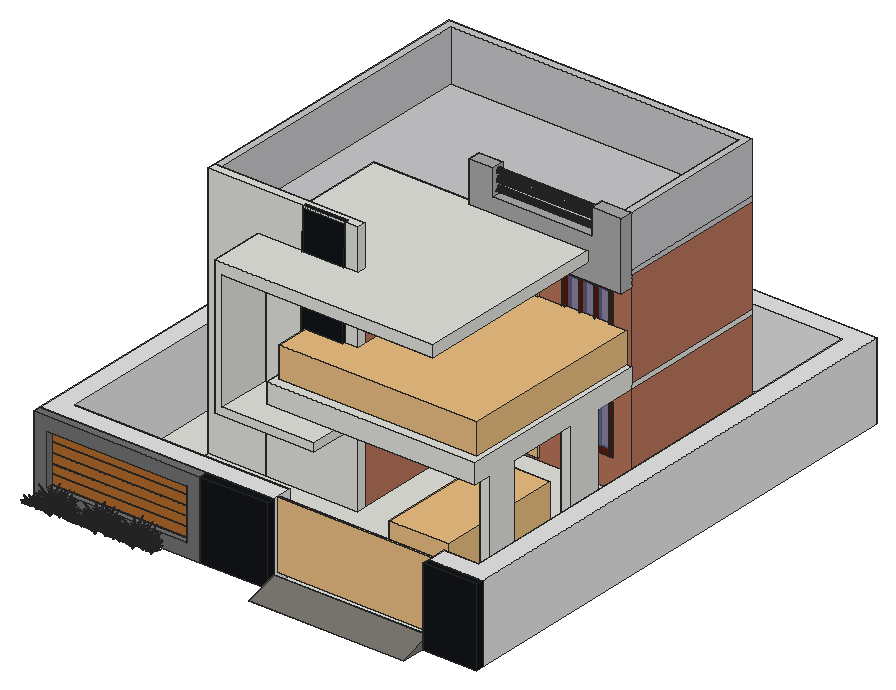
# SketchUp Ruby script. Lengths in inches.
U = 1.inch
M = Sketchup.active_model
def pt(a) = Geom::Point3d.new(a.map { |v| v * U })
def face(e, loops, mat)
  f = e.add_face(loops[0].map { |a| pt(a) })
  loops[1..].each { |l| e.add_face(l.map { |a| pt(a) }).erase! }
  f.material = f.back_material = mat if mat
  f
end
# faces: each face lists its corners as indices into pts; further lists are holes
def faces(e, pts, list, mat = nil) = list.each { |f| face(e, (f[0].is_a?(Array) ? f : [f]).map { |l| l.map { |i| pts[i] } }, mat) }
# xy, xz, yz: faces in a plane at the given z, y or x. An outline is a flat list of corners, or four numbers for a rectangle; further outlines are holes
def ring(l) = l.size == 4 ? [[l[0], l[1]], [l[2], l[1]], [l[2], l[3]], [l[0], l[3]]] : l.each_slice(2).to_a
def flat(e, list, mat, &to3) = list.each { |f| face(e, (f[0].is_a?(Array) ? f : [f]).map { |l| ring(l).map { |u, v| to3.(u, v) } }, mat) }
def xy(e, z, list, mat = nil) = flat(e, list, mat) { |x, y| [x, y, z] }
def xz(e, y, list, mat = nil) = flat(e, list, mat) { |x, z| [x, y, z] }
def yz(e, x, list, mat = nil) = flat(e, list, mat) { |y, z| [x, y, z] }
def lines(e, pts, list) = list.each { |a, b| e.add_line(pt(pts[a]), pt(pts[b])) }
# prism: a flat outline (further loops are holes) pulled along v
def prism(e, loops, v, mat = nil)
  f = face(e, loops, mat); d = Geom::Vector3d.new(v.map { |x| x * U })
  f.pushpull(f.normal.samedirection?(d) ? d.length : -d.length)
end
def box(e, o, s, mat = nil) = prism(e, [[o, [o[0] + s[0], o[1], o[2]], [o[0] + s[0], o[1] + s[1], o[2]], [o[0], o[1] + s[1], o[2]]]], [0, 0, s[2]], mat)
def at(x, y, z, deg = 0) = Geom::Transformation.translation(pt([x, y, z])) * Geom::Transformation.rotation(ORIGIN, Z_AXIS, deg.degrees)
def axes(o, x, y, z) = Geom::Transformation.new([*x, 0, *y, 0, *z, 0, *pt(o).to_a, 1])
def part(name) = M.definitions.add(name)
# library, detail: a bought-in or finely detailed component or shape, given as its bounding box
def library(name, o, s) = part(name).tap { |d| box(d.entities, o, s) }
def detail(e, o, s) = box(e.add_group.entities, o, s)
def put(e, d, t, mat = nil) = e.add_instance(d, t).tap { |i| i.material = mat if mat }
def group(e, t, mat = nil) = e.add_group.tap { |g| g.transformation = t; g.material = mat if mat }.entities
root = M.entities
M.materials.add("Teddy_HairLight").color = [51, 36, 26]
M.materials.add("[Color B08]").color = [102, 25, 0]
M.materials.add("[Color M03]").color = [170, 170, 170]
M.materials.add("[Color M05]").color = [114, 114, 114]
M.materials.add("[Color M08]").color = [30, 30, 30]
M.materials.add("[Iris]").color = [93, 63, 112]
M.materials.add("[Metal Rusted]").color = [184, 117, 91]
M.materials.add("[Polished Concrete New]").color = [200, 200, 203]
M.materials.add("[Polished Concrete Old]").color = [229, 229, 229]
M.materials.add("[Rough Square Concrete Block]").color = [123, 120, 113]
M.materials.add("[Stone Coursed Rough]").color = [19, 22, 25]
M.materials.add("[Translucent Glass Blue]").color = [100, 149, 237]
M.materials["[Translucent Glass Blue]"].alpha = 0.5
M.materials.add("[Wood Bamboo]").color = [177, 105, 43]
M.materials.add("[Wood Veneer 01]").color = [120, 70, 37]
c1 = library("Passenger sedan",[0.01,0.03,0.02],[16.17,34.46,10.62])
c2 = library("Untitled",[332.1875,126.3,0],[192,3,60])
c3 = part("Group\#23")
p = [[2.875,6.8,1.42],[2.44,3.34,0.98],[2.875,0,0],[3.31,3.34,0.98],[2.875,82.68,0],[2.44,79.33,0.98],
  [2.875,75.875,1.42],[3.31,79.33,0.98],[2,6.6875,1.96],[3.74,6.6875,1.96],[2,75.99,1.96],[3.74,75.99,1.96],
  [1.64,10.09,2.76],[4.09,10.09,2.76],[2.875,13.65,2.58],[1.64,72.59,2.76],[2.875,69.03,2.58],[4.09,72.59,2.76],
  [1.29,13.48,3.57],[4.44,13.49,3.57],[1,16.93,4.2],[4.72,16.93,4.2],[2.875,20.54,3.48],[1,65.75,4.2],
  [2.875,62.14,3.48],[4.72,65.75,4.2],[4.44,69.19,3.57],[1.29,69.19,3.57],[0.72,20.37,4.82],[5,20.37,4.82],
  [0.52,23.85,5.28],[5.19,23.85,5.28],[2.875,27.46,4.13],[0.52,58.83,5.28],[2.875,55.22,4.13],[5.19,58.83,5.28],
  [0.72,62.31,4.82],[5,62.31,4.82],[0.32,27.32,5.73],[5.39,27.32,5.73],[0.2,30.82,6],[5.51,30.82,6],
  [2.875,34.39,4.52],[0.2,51.86,6],[2.875,48.28,4.52],[5.51,51.86,6],[0.32,55.35,5.73],[5.39,55.35,5.73],
  [0.08,34.32,6.27],[5.63,34.32,6.27],[0.04,37.83,6.36],[5.67,37.83,6.36],[2.875,41.34,4.65],[0.04,44.85,6.36],
  [5.67,44.85,6.36],[0.08,48.36,6.27],[5.63,48.36,6.27],[0,41.34,6.45],[5.71,41.34,6.45]]
faces(c3.entities,p,[[0,1,2],[3,0,2],[4,5,6],[7,4,6],[0,8,1],[9,0,3],[6,5,10],[11,7,6],
  [0,12,8],[13,0,9],[14,12,0],[13,14,0],[6,15,16],[17,6,16],[6,10,15],[17,11,6],
  [14,18,12],[19,14,13],[14,20,18],[21,14,19],[22,20,14],[21,22,14],[16,23,24],[25,16,24],
  [25,26,16],[16,27,23],[16,15,27],[26,17,16],[22,28,20],[29,22,21],[22,30,28],[31,22,29],
  [32,30,22],[31,32,22],[24,33,34],[35,24,34],[24,36,33],[35,37,24],[24,23,36],[37,25,24],
  [32,38,30],[39,32,31],[32,40,38],[41,32,39],[42,40,32],[41,42,32],[34,43,44],[45,34,44],
  [34,46,43],[45,47,34],[34,33,46],[47,35,34],[42,48,40],[49,42,41],[42,50,48],[51,42,49],
  [52,50,42],[51,52,42],[44,53,52],[54,44,52],[44,55,53],[54,56,44],[44,43,55],[56,45,44],
  [52,57,50],[58,52,51],[52,53,57],[58,54,52]],"[Iris]")
c4 = part("Group\#25")
put(c4.entities,c3,axes([28.08,0,71.6],[1,0,0],[0,0.5,-0.86603],[0,0.86603,0.5]))
put(c4.entities,c3,axes([2.85,59.63,58],[-0.405,-0.70148,0],[0.35074,-0.2025,-0.70148],[0.6075,-0.35074,0.405]))
put(c4.entities,c3,axes([-1.6,23.09,64.44],[0.55484,-0.83195,0],[0.37438,0.24968,-0.77942],[0.72049,0.48051,0.5]))
c5 = part("Group\#26")
put(c5.entities,c3,axes([28.08,0,71.6],[1,0,0],[0,0.5,-0.86603],[0,0.86603,0.5]))
put(c5.entities,c3,axes([2.85,59.63,58],[-0.405,-0.70148,0],[0.35074,-0.2025,-0.70148],[0.6075,-0.35074,0.405]))
put(c5.entities,c3,axes([-1.6,23.09,64.44],[0.55484,-0.83195,0],[0.37438,0.24968,-0.77942],[0.72049,0.48051,0.5]))
c6 = part("Group\#28")
put(c6.entities,c4,at(0.8125,72.29,3.66,-90))
put(c6.entities,c5,at(11.2,0,3.66))
put(c6.entities,c5,axes([83.03,10.65,3.66],[0,1,0],[-1,0,0],[0,0,0.6674]))
put(c6.entities,c4,axes([10.73,0.27,3.66],[1,0,0],[0,1,0],[0,0,0.6674]))
put(c6.entities,c4,axes([0,74.01,0],[0,-1,0],[1,0,0],[0,0,0.6674]))
put(c6.entities,c5,axes([10.39,1.72,0],[1,0,0],[0,1,0],[0,0,0.6674]))
c7 = part("Group\#27")
put(c7.entities,c4,at(0.8125,72.29,3.66,-90))
g1 = group(c7.entities,at(11.2,0,3.66))
put(g1,c3,axes([28.08,0,71.6],[1,0,0],[0,0.5,-0.86603],[0,0.86603,0.5]))
put(g1,c3,axes([2.85,59.63,58],[-0.405,-0.70148,0],[0.35074,-0.2025,-0.70148],[0.6075,-0.35074,0.405]))
put(g1,c3,axes([-1.6,23.09,64.44],[0.55484,-0.83195,0],[0.37438,0.24968,-0.77942],[0.72049,0.48051,0.5]))
put(c7.entities,c5,axes([83.03,10.65,3.66],[0,1,0],[-1,0,0],[0,0,0.6674]))
put(c7.entities,c4,axes([10.73,0.27,3.66],[1,0,0],[0,1,0],[0,0,0.6674]))
put(c7.entities,c4,axes([0,74.01,0],[0,-1,0],[1,0,0],[0,0,0.6674]))
put(c7.entities,c5,axes([10.39,1.72,0],[1,0,0],[0,1,0],[0,0,0.6674]))
c8 = part("3D MAGUEY MORADO\#1")
g2 = group(c8.entities,at(-32.99,-10.27,-0.83))
put(g2,c6,axes([-39.6875,16.46,0],[0.24592,-0.0659,0],[0.0659,0.24592,0],[0,0,0.11838]))
put(g2,c6,axes([-26.5,33.58,0],[0.24592,-0.0659,0],[-0.0659,-0.24592,0],[0,0,0.11726]))
put(g2,c6,axes([-17.68,35.06,0],[0.24592,-0.0659,0],[-0.0659,-0.24592,0],[0,0,0.11629]))
put(g2,c6,axes([-10.91,34.03,0],[0.24592,-0.0659,0],[-0.0659,-0.24592,0],[0,0,0.08614]))
put(g2,c6,axes([-42.47,34.03,0],[0.24592,-0.0659,0],[-0.0659,-0.24592,0],[0,0,0.11358]))
put(g2,c6,axes([-35.12,28.93,1.27],[0.24592,-0.0659,0],[-0.0659,-0.24592,0],[0,0,0.13496]))
put(g2,c6,axes([-21.65,27.42,0],[0.24592,-0.0659,0],[-0.0659,-0.24592,0],[0,0,0.04307]))
put(g2,c6,axes([-59.75,22.9375,0],[0.19331,0.16569,0],[0.16569,-0.19331,0],[0,0,0.10473]))
put(g2,c6,axes([-33.52,38.94,0],[0.32359,-0.0867,0],[-0.0867,-0.32359,0],[0,0,0.1288]))
put(g2,c6,axes([-32.6875,6.24,0],[0.32359,-0.0867,0],[0.0867,0.32359,0],[0,0,0.1288]))
put(g2,c7,axes([-6.69,0,0],[0,0.335,0],[-0.335,0,0],[0,0,0.17889]))
put(g2,c7,axes([-19.43,3.43,0],[0,0.335,0],[-0.335,0,0],[0,0,0.17889]))
put(g2,c7,axes([-26.35,6.74,0.74],[0,0.335,0],[-0.335,0,0],[0,0,0.17889]))
c9 = part("Group3\#1")
xy(c9.entities,0,[[-27.28,-27.28,-9.89,27.28],[-8.7,-27.28,8.7,27.28],[9.89,-27.28,27.28,27.28]],"[Translucent Glass Blue]")
c10 = part("Group2\#1")
xy(c10.entities,0,[[[-31.22,-31.22,31.22,31.22],[-8.7,-27.28,8.7,27.28],[9.89,-27.28,27.28,27.28],[-27.28,-27.28,-9.89,27.28]]],"[Wood Veneer 01]")
xy(c10.entities,10,[[[-31.22,-31.22,31.22,31.22],[-8.7,-27.28,8.7,27.28],[9.89,-27.28,27.28,27.28],[-27.28,-27.28,-9.89,27.28]]],"[Color B08]")
xz(c10.entities,-31.22,[[-31.22,0,31.22,10]],"[Wood Veneer 01]")
xz(c10.entities,-27.28,[[-27.28,0,-9.89,10],[-8.7,0,8.7,10],[9.89,0,27.28,10]],"[Color B08]")
xz(c10.entities,27.28,[[-27.28,0,-9.89,10],[-8.7,0,8.7,10],[9.89,0,27.28,10]],"[Color B08]")
xz(c10.entities,31.22,[[-31.22,0,31.22,10]],"[Wood Veneer 01]")
yz(c10.entities,-31.22,[[-31.22,0,31.22,10]],"[Wood Veneer 01]")
yz(c10.entities,-27.28,[[-27.28,0,27.28,10]],"[Color B08]")
yz(c10.entities,-9.89,[[-27.28,0,27.28,10]],"[Color B08]")
yz(c10.entities,-8.7,[[-27.28,0,27.28,10]],"[Wood Veneer 01]")
yz(c10.entities,8.7,[[-27.28,0,27.28,10]],"[Color B08]")
yz(c10.entities,9.89,[[-27.28,0,27.28,10]],"[Wood Veneer 01]")
yz(c10.entities,27.28,[[-27.28,0,27.28,10]],"[Color B08]")
yz(c10.entities,31.22,[[-31.22,0,31.22,10]],"[Wood Veneer 01]")
put(c10.entities,c9,at(0,0,5),"[Color B08]")
c11 = library("Group\#1",[0,0,0],[52.38,10.47,93])
c12 = part("Group1\#2")
xy(c12.entities,0,[[[138.0625,174.875,138.0625,537.875,513.0625,537.875,513.0625,351.875,324.0625,351.875,324.0625,174.875],[147.0625,183.875,315.0625,183.875,315.0625,360.875,504.0625,360.875,504.0625,528.875,147.0625,528.875]]],"[Metal Rusted]")
xy(c12.entities,3,[[345.36,351.875,397.74,360.875]],"[Metal Rusted]")
xy(c12.entities,96,[[345.36,351.875,397.74,360.875]],"[Metal Rusted]")
xy(c12.entities,120,[[[138.0625,174.875,324.0625,174.875,324.0625,351.875,513.0625,351.875,513.0625,537.875,138.0625,537.875],[147.0625,183.875,147.0625,528.875,504.0625,528.875,504.0625,360.875,315.0625,360.875,315.0625,183.875]]],"[Metal Rusted]")
xz(c12.entities,174.875,[[138.0625,0,324.0625,120]],"[Metal Rusted]")
xz(c12.entities,183.875,[[147.0625,0,315.0625,120]],"[Metal Rusted]")
xz(c12.entities,351.875,[[[324.0625,0,513.0625,120],[345.36,3,397.74,96],[426.53,34.52,488.96,96.96]]],"[Metal Rusted]")
xz(c12.entities,360.875,[[[315.0625,0,504.0625,120],[345.36,3,397.74,96]]],"[Metal Rusted]")
xz(c12.entities,528.875,[[147.0625,0,504.0625,120]],"[Metal Rusted]")
xz(c12.entities,537.875,[[138.0625,0,513.0625,120]],"[Metal Rusted]")
yz(c12.entities,138.0625,[[174.875,0,537.875,120]],"[Metal Rusted]")
yz(c12.entities,147.0625,[[183.875,0,528.875,120]],"[Metal Rusted]")
yz(c12.entities,315.0625,[[183.875,0,360.875,120]],"[Metal Rusted]")
yz(c12.entities,324.0625,[[174.875,0,351.875,120]],"[Metal Rusted]")
yz(c12.entities,345.36,[[351.875,3,360.875,96]],"[Metal Rusted]")
yz(c12.entities,397.74,[[351.875,3,360.875,96]],"[Metal Rusted]")
yz(c12.entities,504.0625,[[360.875,0,528.875,120]],"[Metal Rusted]")
yz(c12.entities,513.0625,[[351.875,0,537.875,120]],"[Metal Rusted]")
put(c12.entities,c10,axes([457.75,361.875,65.74],[1,0,0],[0,0,1],[0,-1,0]))
put(c12.entities,c11,at(345.36,350.4,3))
c13 = part("Group2\#2")
xy(c13.entities,0,[[[-31.22,-31.22,31.22,31.22],[-8.7,-27.28,8.7,27.28],[9.89,-27.28,27.28,27.28],[-27.28,-27.28,-9.89,27.28]]],"[Wood Veneer 01]")
xy(c13.entities,10,[[[-31.22,-31.22,31.22,31.22],[-8.7,-27.28,8.7,27.28],[9.89,-27.28,27.28,27.28],[-27.28,-27.28,-9.89,27.28]]],"[Color B08]")
xz(c13.entities,-31.22,[[-31.22,0,31.22,10]],"[Wood Veneer 01]")
xz(c13.entities,-27.28,[[-27.28,0,-9.89,10],[-8.7,0,8.7,10],[9.89,0,27.28,10]],"[Color B08]")
xz(c13.entities,27.28,[[-27.28,0,-9.89,10],[-8.7,0,8.7,10],[9.89,0,27.28,10]],"[Color B08]")
xz(c13.entities,31.22,[[-31.22,0,31.22,10]],"[Wood Veneer 01]")
yz(c13.entities,-31.22,[[-31.22,0,31.22,10]],"[Wood Veneer 01]")
yz(c13.entities,-27.28,[[-27.28,0,27.28,10]],"[Color B08]")
yz(c13.entities,-9.89,[[-27.28,0,27.28,10]],"[Color B08]")
yz(c13.entities,-8.7,[[-27.28,0,27.28,10]],"[Color B08]")
yz(c13.entities,8.7,[[-27.28,0,27.28,10]],"[Color B08]")
yz(c13.entities,9.89,[[-27.28,0,27.28,10]],"[Color B08]")
yz(c13.entities,27.28,[[-27.28,0,27.28,10]],"[Color B08]")
yz(c13.entities,31.22,[[-31.22,0,31.22,10]],"[Wood Veneer 01]")
put(c13.entities,c9,at(0,0,5),"[Wood Veneer 01]")
c14 = library("Group\#10",[0,0,0],[52.38,10.47,93])
c15 = part("Group1\#1")
xy(c15.entities,0,[[[138.0625,174.875,138.0625,537.875,513.0625,537.875,513.0625,351.875,324.0625,351.875,324.0625,174.875],[147.0625,183.875,315.0625,183.875,315.0625,360.875,504.0625,360.875,504.0625,528.875,147.0625,528.875]]])
xy(c15.entities,3,[[345.36,351.875,397.74,360.875]])
xy(c15.entities,96,[[345.36,351.875,397.74,360.875]])
xy(c15.entities,120,[[[138.0625,174.875,324.0625,174.875,324.0625,351.875,513.0625,351.875,513.0625,537.875,138.0625,537.875],[147.0625,183.875,147.0625,528.875,504.0625,528.875,504.0625,360.875,315.0625,360.875,315.0625,183.875]]])
xz(c15.entities,174.875,[[138.0625,0,324.0625,120]])
xz(c15.entities,183.875,[[147.0625,0,315.0625,120]])
xz(c15.entities,351.875,[[[324.0625,0,513.0625,120],[345.36,3,397.74,96],[426.53,34.52,488.96,96.96]]])
xz(c15.entities,360.875,[[[315.0625,0,504.0625,120],[345.36,3,397.74,96]]])
xz(c15.entities,528.875,[[147.0625,0,504.0625,120]])
xz(c15.entities,537.875,[[138.0625,0,513.0625,120]])
yz(c15.entities,138.0625,[[174.875,0,537.875,120]])
yz(c15.entities,147.0625,[[183.875,0,528.875,120]])
yz(c15.entities,315.0625,[[183.875,0,360.875,120]])
yz(c15.entities,324.0625,[[174.875,0,351.875,120]])
yz(c15.entities,345.36,[[351.875,3,360.875,96]])
yz(c15.entities,397.74,[[351.875,3,360.875,96]])
yz(c15.entities,504.0625,[[360.875,0,528.875,120]])
yz(c15.entities,513.0625,[[351.875,0,537.875,120]])
put(c15.entities,c13,axes([457.75,361.875,65.74],[1,0,0],[0,0,1],[0,-1,0]))
put(c15.entities,c14,at(345.36,350.4,3))
c16 = library("Group\#14",[0,0,0],[244.71,233.92,37.74])
c17 = part("Group24\#1")
prism(c17.entities,[[[504.0625,528.875,252],[147.0625,528.875,252],[147.0625,174.875,252],[138.0625,174.875,252],[138.0625,537.875,252],[513.0625,537.875,252],[513.0625,351.875,252],[504.0625,351.875,252]]],[0,0,63.75])
c18 = part("Group71\#1")
xy(c18.entities,9.55,[[1128.23,1998.9,1301.9,1999.9],[1128.23,1999.9,1301.9,2031.65]],"[Wood Bamboo]")
xy(c18.entities,10.55,[[1128.23,1998.9,1301.9,1999.9]],"[Wood Bamboo]")
xy(c18.entities,21.36,[[1128.23,1998.9,1301.9,1999.9]],"[Wood Bamboo]")
xy(c18.entities,22.36,[[1128.23,1998.9,1301.9,1999.9]],"[Wood Bamboo]")
xy(c18.entities,33.17,[[1128.23,1998.9,1301.9,1999.9]],"[Wood Bamboo]")
xy(c18.entities,34.17,[[1128.23,1998.9,1301.9,1999.9]],"[Wood Bamboo]")
xy(c18.entities,44.98,[[1128.23,1998.9,1301.9,1999.9]],"[Wood Bamboo]")
xy(c18.entities,45.98,[[1128.23,1998.9,1301.9,1999.9]],"[Wood Bamboo]")
xy(c18.entities,56.8,[[1128.23,1998.9,1301.9,1999.9]],"[Wood Bamboo]")
xy(c18.entities,57.8,[[1128.23,1998.9,1301.9,1999.9]],"[Wood Bamboo]")
xy(c18.entities,72.51,[[1128.23,1998.9,1301.9,2031.65]],"[Wood Bamboo]")
xz(c18.entities,1998.9,[[1128.23,10.55,1301.9,21.36],[1128.23,22.36,1301.9,33.17],[1128.23,34.17,1301.9,44.98],[1128.23,45.98,1301.9,56.8],[1128.23,57.8,1301.9,72.51]],"[Wood Bamboo]")
xz(c18.entities,1999.9,[[1128.23,9.55,1301.9,10.55],[1128.23,21.36,1301.9,22.36],[1128.23,33.17,1301.9,34.17],[1128.23,44.98,1301.9,45.98],[1128.23,56.8,1301.9,57.8]],"[Wood Bamboo]")
xz(c18.entities,2031.65,[[1128.23,9.55,1301.9,72.51]],"[Wood Bamboo]")
yz(c18.entities,1128.23,[[1998.9,9.55,1999.9,10.55],[1999.9,9.55,1999.9,10.55,1998.9,10.55,1998.9,21.36,1999.9,21.36,1999.9,22.36,1998.9,22.36,1998.9,33.17,1999.9,33.17,1999.9,34.17,1998.9,34.17,1998.9,44.98,1999.9,44.98,1999.9,45.98,1998.9,45.98,1998.9,56.8,1999.9,56.8,1999.9,57.8,1998.9,57.8,1998.9,72.51,2031.65,72.51,2031.65,9.55],[1998.9,21.36,1999.9,22.36],[1998.9,33.17,1999.9,34.17],[1998.9,44.98,1999.9,45.98],
  [1998.9,56.8,1999.9,57.8]],"[Wood Bamboo]")
yz(c18.entities,1301.9,[[1998.9,9.55,1999.9,10.55],[1999.9,9.55,2031.65,9.55,2031.65,72.51,1998.9,72.51,1998.9,57.8,1999.9,57.8,1999.9,56.8,1998.9,56.8,1998.9,45.98,1999.9,45.98,1999.9,44.98,1998.9,44.98,1998.9,34.17,1999.9,34.17,1999.9,33.17,1998.9,33.17,1998.9,22.36,1999.9,22.36,1999.9,21.36,1998.9,21.36,1998.9,10.55,1999.9,10.55],[1998.9,21.36,1999.9,22.36],[1998.9,33.17,1999.9,34.17],[1998.9,44.98,1999.9,45.98],
  [1998.9,56.8,1999.9,57.8]],"[Wood Bamboo]")
g3 = group(c18.entities,at(1111.71,2000.75,-6.97))
prism(g3,[[[521.94,588.78,0],[24,588.78,0],[24,24.09,0],[289.9375,24.09,0],[289.9375,0.09,0],[0,0.09,0],[0,612.78,0],[545.85,612.78,0],[548.12,0.09,0],[481.81,-0.16,0],[481.72,23.84,0],[524.03,24,0]]],[0,0,96])
prism(root,[[[481.81,43.57,-6.97],[548.12,43.82,-6.97],[548.16,34.77,-6.97],[481.84,34.53,-6.97]]],[0,0,96],"[Stone Coursed Rough]")
xy(root,-6.97,[[206.7,33.82,289.9375,43.82],[[0,43.82,545.85,656.5],[84,127.82,459,572.5]],[84,127.82,459,572.5]])
xy(root,-0.97,[[84,127.82,459,572.5]])
xy(root,89.03,[[206.7,33.82,289.9375,43.82]],"[Stone Coursed Rough]")
xy(root,95.3125,[[146.82,131.07,270,209.5]])
xy(root,105.28,[[156.03,131.07,270,209.5]])
xy(root,252,[[156.03,131.07,156.03,209.5,146.82,209.5,146.82,376.88,416.9,376.88,416.9,131.07]])
xy(root,265.95,[[146.82,131.07,416.9,376.88]])
xz(root,33.82,[[206.7,-6.97,289.9375,89.03]],"[Stone Coursed Rough]")
xz(root,43.82,[[206.7,-6.97,289.9375,89.03]])
xz(root,127.82,[[84,-6.97,459,-0.97]])
xz(root,131.07,[[146.82,95.3125,270,95.3125,270,105.28,156.03,105.28,156.03,252,416.9,252,416.9,265.95,146.82,265.95]])
xz(root,209.5,[[146.82,95.3125,146.82,252,156.03,252,156.03,105.28,270,105.28,270,95.3125]])
xz(root,376.88,[[146.82,252,416.9,265.95]])
xz(root,572.5,[[84,-6.97,459,-0.97]])
yz(root,84,[[127.82,-6.97,572.5,-0.97]])
yz(root,146.82,[[131.07,95.3125,131.07,265.95,376.88,265.95,376.88,252,209.5,252,209.5,95.3125]])
yz(root,156.03,[[131.07,105.28,202.94,252],[202.94,105.28,209.5,252]])
yz(root,206.7,[[33.82,-6.97,43.82,89.03]],"[Stone Coursed Rough]")
yz(root,270,[[131.07,95.3125,202.94,105.28],[202.94,95.3125,209.5,105.28]])
yz(root,289.9375,[[33.82,-6.97,43.82,89.03]],"[Stone Coursed Rough]")
yz(root,416.9,[[131.07,252,376.88,265.95]])
yz(root,459,[[127.82,-6.97,572.5,-0.97]])
put(root,c1,axes([431.44,294.99,-0.57],[-4.53288,0,0],[0,-4.57821,0],[0,0,4.53288]))
put(root,c2,axes([-42.44,-103.55,6.2],[1.00009,0,0],[0,1.19874,0],[0,0,1.38057]))
put(root,c8,axes([-28.52,25.02,-2.3],[-1.13,0,0],[0,-1,0],[0,0,1.69568]))
put(root,c8,axes([27.54,25.02,-2.3],[-1.13,0,0],[0,-1,0],[0,0,1.69568]))
put(root,c8,axes([74.29,25.02,-2.3],[-1.13,0,0],[0,-1,0],[0,0,1.69568]))
put(root,c12,at(-54.0625,34.63,0))
g4 = group(root,at(84,209.5,120))
prism(g4,[[[0,0,0],[0,363,0],[375,363,0],[375,177,0],[186,177,0],[186,0,0]]],[0,0,6])
put(root,c15,at(-54.0625,34.63,126),"[Metal Rusted]")
g5 = group(root,at(270,386.5,120))
xy(g5,-120.97,[[176.9375,-219.75,189,-182.625]])
xy(g5,-120,[[176.9375,-94.6875,189,-52.0625]])
xy(g5,0,[[-68.1875,-243.625,-68.1875,0,189,0,189,-52.0625,176.9375,-52.0625,176.9375,-94.6875,189,-94.6875,189,-182.625,176.9375,-182.625,176.9375,-219.75,189,-219.75,189,-243.625]])
xy(g5,24.8125,[[-68.1875,-243.625,189,0]])
xz(g5,-243.625,[[-68.1875,0,189,24.8125]])
xz(g5,-219.75,[[176.9375,-120.97,189,0]])
xz(g5,-182.625,[[176.9375,-120.97,189,0]])
xz(g5,-94.6875,[[176.9375,-120,189,0]])
xz(g5,-52.0625,[[176.9375,-120,189,0]])
xz(g5,0,[[-68.1875,0,189,24.8125]])
yz(g5,-68.1875,[[-243.625,0,0,24.8125]])
yz(g5,176.9375,[[-219.75,-120.97,-182.625,0],[-94.6875,-120,-52.0625,0]])
yz(g5,189,[[-219.75,-120.97,-182.625,-120.97,-182.625,0,-94.6875,0,-94.6875,-120,-52.0625,-120,-52.0625,0,0,0,0,24.8125,-243.625,24.8125,-243.625,0,-219.75,0]])
put(g5,c16,at(-61.99,-231.95,24.8125))
g6 = group(root,at(84,209.5,246),"[Polished Concrete New]")
prism(g6,[[[0,0,0],[0,363,0],[375,363,0],[375,177,0],[186,177,0],[186,0,0]]],[0,0,6])
put(g6,c17,at(-138.0625,-174.875,-246))
g7 = group(root,at(270,386.5,232.15),"[Color M03]")
prism(g7,[[[29.48,-16.1875,83.6],[0,-16.1875,83.6],[0,-16.1875,0],[189,-16.1875,0],[189,-16.1875,83.6],[152.3,-16.1875,83.6],[152.3,-16.1875,51.41],[29.48,-16.1875,51.41]]],[0,16.1875,0])
p = [[189,-16.1875,83.6],[189,-16.625,83.6],[0,-16.1875,0],[0,-16.625,0],[189,-16.1875,0],[189,-16.625,0],
  [0,-16.1875,83.6],[0,-16.625,83.6]]
lines(g7,p,[[0,1],[2,3],[4,5],[6,7]])
g8 = group(g7,at(29.48,-10.9,75.15),"[Color M08]")
prism(g8,[[[0,1.47,0.39],[0,0.86,0.86],[0,0.39,1.47],[0,0.1,2.18],[0,0,2.9375],[0,0.1,3.7],[0,0.39,4.41],[0,0.86,5.01],[0,1.47,5.48],[0,2.18,5.77],[0,2.9375,5.875],[0,3.7,5.77],[0,4.41,5.48],[0,5.01,5.01],[0,5.48,4.41],[0,5.77,3.7],[0,5.875,2.9375],[0,5.77,2.18],[0,5.48,1.47],[0,5.01,0.86],[0,4.41,0.39],[0,3.7,0.1],[0,2.9375,0],[0,2.18,0.1]]],[122.8125,0,0])
g9 = group(g7,at(29.48,-10.9,65.65),"[Color M08]")
prism(g9,[[[0,1.47,0.39],[0,0.86,0.86],[0,0.39,1.47],[0,0.1,2.18],[0,0,2.9375],[0,0.1,3.7],[0,0.39,4.41],[0,0.86,5.01],[0,1.47,5.48],[0,2.18,5.77],[0,2.9375,5.875],[0,3.7,5.77],[0,4.41,5.48],[0,5.01,5.01],[0,5.48,4.41],[0,5.77,3.7],[0,5.875,2.9375],[0,5.77,2.18],[0,5.48,1.47],[0,5.01,0.86],[0,4.41,0.39],[0,3.7,0.1],[0,2.9375,0],[0,2.18,0.1]]],[122.8125,0,0])
g10 = group(g7,at(29.48,-10.9,55.09),"[Color M08]")
prism(g10,[[[0,1.47,0.39],[0,0.86,0.86],[0,0.39,1.47],[0,0.1,2.18],[0,0,2.9375],[0,0.1,3.7],[0,0.39,4.41],[0,0.86,5.01],[0,1.47,5.48],[0,2.18,5.77],[0,2.9375,5.875],[0,3.7,5.77],[0,4.41,5.48],[0,5.01,5.01],[0,5.48,4.41],[0,5.77,3.7],[0,5.875,2.9375],[0,5.77,2.18],[0,5.48,1.47],[0,5.01,0.86],[0,4.41,0.39],[0,3.7,0.1],[0,2.9375,0],[0,2.18,0.1]]],[122.8125,0,0])
g11 = group(root,at(84,209.5,0))
box(g11,[0,-11.0625,0],[186,11.0625,315.75])
g12 = group(root,at(156.03,202.94,0))
prism(g12,[[[0,0,252],[113.97,0,252],[113.97,0,105.28],[113.97,0,95.3125],[113.97,0,0],[0,0,0],[0,0,105.28]]],[0,-4.8125,0])
g13 = group(root,at(202.58,198.13,145.46),"Teddy_HairLight")
g14 = group(g13,at(0,-4.4375,0),"[Stone Coursed Rough]")
prism(g14,[[[0,4.4375,0],[51.49,4.4375,0],[51.49,0,0.125],[0,0,0.125]]],[0,4.8125,170.29])
put(root,c18,at(-1111.71,-1957.02,0),"[Polished Concrete Old]")
g15 = group(root,at(289.9375,5.63,-6.97),"[Rough Square Concrete Block]")
xy(g15,0,[[0,0,191.48,38.18]])
xz(g15,38.18,[[0,0,0.375,12,191.86,12,191.48,0]])
p = [[0.375,38.18,12],[0,0,0],[191.48,0,0],[191.86,38.18,12],[0,38.18,0],[191.48,38.18,0]]
faces(g15,p,[[0,1,2,3],[4,1,0],[2,5,3]])
g16 = group(root,at(0,43.82,-6.97))
prism(g16,[[[0,-10,0],[206.7,-10,0],[206.7,-10,96],[0,-10,96]],[[190.1875,-10,16.52],[16.52,-10,16.52],[16.52,-10,79.48],[190.1875,-10,79.48]]],[0,10,0],"[Color M05]")
